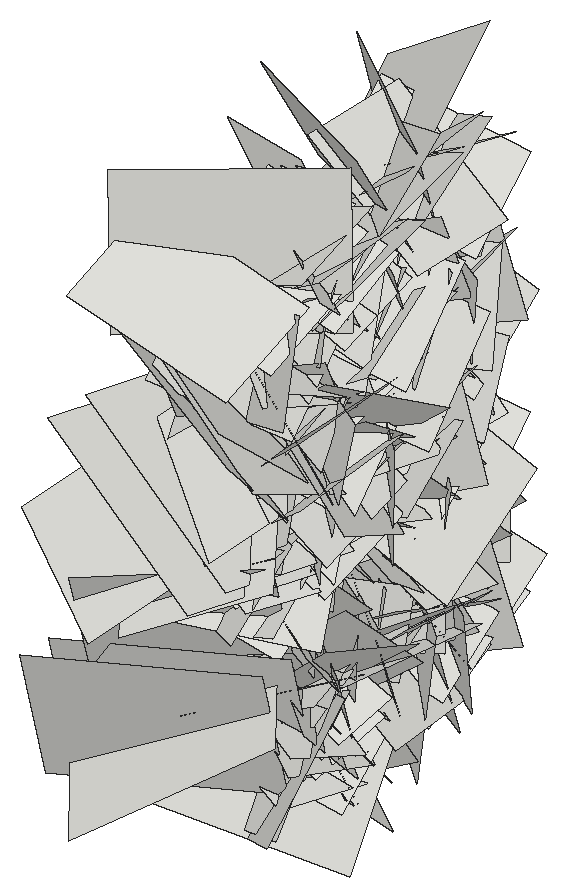
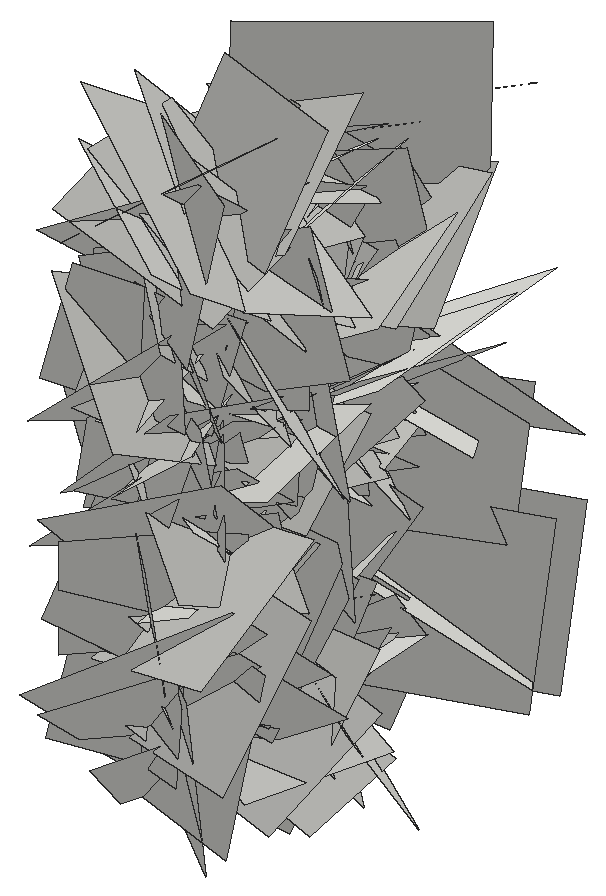
# SketchUp Ruby script. Lengths in inches.
U = 1.inch
M = Sketchup.active_model
def pt(a) = Geom::Point3d.new(a.map { |v| v * U })
def face(e, loops, mat)
  f = e.add_face(loops[0].map { |a| pt(a) })
  loops[1..].each { |l| e.add_face(l.map { |a| pt(a) }).erase! }
  f.material = f.back_material = mat if mat
  f
end
# faces: each face lists its corners as indices into pts; further lists are holes
def faces(e, pts, list, mat = nil) = list.each { |f| face(e, (f[0].is_a?(Array) ? f : [f]).map { |l| l.map { |i| pts[i] } }, mat) }
# xy, xz, yz: faces in a plane at the given z, y or x. An outline is a flat list of corners, or four numbers for a rectangle; further outlines are holes
def ring(l) = l.size == 4 ? [[l[0], l[1]], [l[2], l[1]], [l[2], l[3]], [l[0], l[3]]] : l.each_slice(2).to_a
def flat(e, list, mat, &to3) = list.each { |f| face(e, (f[0].is_a?(Array) ? f : [f]).map { |l| ring(l).map { |u, v| to3.(u, v) } }, mat) }
def xy(e, z, list, mat = nil) = flat(e, list, mat) { |x, y| [x, y, z] }
def xz(e, y, list, mat = nil) = flat(e, list, mat) { |x, z| [x, y, z] }
def yz(e, x, list, mat = nil) = flat(e, list, mat) { |y, z| [x, y, z] }
def lines(e, pts, list) = list.each { |a, b| e.add_line(pt(pts[a]), pt(pts[b])) }
# prism: a flat outline (further loops are holes) pulled along v
def prism(e, loops, v, mat = nil)
  f = face(e, loops, mat); d = Geom::Vector3d.new(v.map { |x| x * U })
  f.pushpull(f.normal.samedirection?(d) ? d.length : -d.length)
end
def box(e, o, s, mat = nil) = prism(e, [[o, [o[0] + s[0], o[1], o[2]], [o[0] + s[0], o[1] + s[1], o[2]], [o[0], o[1] + s[1], o[2]]]], [0, 0, s[2]], mat)
def at(x, y, z, deg = 0) = Geom::Transformation.translation(pt([x, y, z])) * Geom::Transformation.rotation(ORIGIN, Z_AXIS, deg.degrees)
def axes(o, x, y, z) = Geom::Transformation.new([*x, 0, *y, 0, *z, 0, *pt(o).to_a, 1])
def part(name) = M.definitions.add(name)
# library, detail: a bought-in or finely detailed component or shape, given as its bounding box
def library(name, o, s) = part(name).tap { |d| box(d.entities, o, s) }
def detail(e, o, s) = box(e.add_group.entities, o, s)
def put(e, d, t, mat = nil) = e.add_instance(d, t).tap { |i| i.material = mat if mat }
def group(e, t, mat = nil) = e.add_group.tap { |g| g.transformation = t; g.material = mat if mat }.entities
root = M.entities
c1 = part("Component\#6")
p = [[0.01,0,0],[0,3.24,4.54],[4.32,3.24,4.54],[4.33,0,0]]
faces(c1.entities,p,[[0,1,2,3]])
put(root,c1,axes([404.99,125.5,13.2],[-1.07209,0.56535,0.5401],[-0.40295,0.41611,-1.14744],[-0.72423,-1.06841,-0.1611]))
put(root,c1,axes([404.88,125.3125,7.6875],[-0.15543,0.49215,-1.26812],[-0.29157,-1.25984,-0.45713],[-1.41209,0.20597,0.23397]))
put(root,c1,axes([404.88,126.76,7.6875],[-0.15543,0.49215,-1.26812],[-0.29157,-1.25984,-0.45713],[-1.41209,0.20597,0.23397]))
put(root,c1,axes([404.88,135.96,3.29],[-0.1622,-0.76384,1.11136],[-0.23079,1.11781,0.7383],[-1.4107,-0.09505,-0.24857]))
put(root,c1,axes([404.88,130.15,15.41],[-0.24379,0.89731,1.03665],[-0.02149,1.04879,-0.91232],[-1.45316,-0.16605,-0.16042]))
put(root,c1,axes([404.88,136.82,5.83],[-0.1656,-1.02965,0.80161],[-0.14776,0.81588,1.02082],[-1.37528,0.03632,-0.2062]))
put(root,c1,axes([404.88,130.78,10.54],[-0.24762,-1.26357,-0.1726],[0.00687,-0.17664,1.28442],[-1.3518,0.23056,0.03815]))
put(root,c1,axes([406.05,124.5,5.79],[-0.83668,1.07369,0.2523],[-0.21003,0.16716,-1.33127],[-1.15009,-0.81162,0.05958]))
put(root,c1,axes([404.88,138.98,4.78],[-0.22268,-0.9196,-0.8307],[-0.07298,-0.83259,0.9391],[-1.31157,0.20246,0.08879]))
put(root,c1,axes([404.88,128.0625,10.23],[-0.10909,-1.3698,0.20566],[0.00727,0.20572,1.37363],[-1.46824,0.1028,-0.00848]))
put(root,c1,axes([404.88,129.98,10.23],[-0.10909,-1.3698,0.20566],[0.00727,0.20572,1.37363],[-1.46824,0.1028,-0.00848]))
put(root,c1,axes([404.88,135.39,1.18],[-0.01455,-0.40823,1.27358],[-0.1801,1.26386,0.40328],[-1.40617,-0.15765,-0.06483]))
put(root,c1,axes([404.88,137,19.49],[-0.23927,-0.1296,-1.18474],[-0.04055,-1.20439,0.13904],[-1.26266,0.06324,0.22004]))
put(root,c1,axes([404.88,127.67,13.74],[-0.06329,-0.97705,0.81505],[-0.12838,0.8166,0.97005],[-1.34259,-0.03203,-0.13118]))
put(root,c1,axes([404.88,125.99,1.35],[-0.00241,0.79041,1.08039],[-0.06651,1.07914,-0.78963],[-1.41741,-0.05198,0.03522]))
put(root,c1,axes([404.88,132.12,7.08],[0.00585,1.22451,-0.43101],[-0.11167,-0.42917,-1.22063],[-1.3715,0.04016,0.09755]))
put(root,c1,axes([404.88,133.15,22.79],[-0.15509,1.06813,0.73269],[0.10614,0.74447,-1.06531],[-1.36888,-0.06329,-0.16562]))
put(root,c1,axes([404.88,128.24,17.68],[-0.22785,0.52614,1.07761],[0.06777,1.09826,-0.52347],[-1.26934,-0.03581,-0.22138]))
put(root,c1,axes([404.88,133.04,19.75],[-0.14526,-0.49923,0.95494],[-0.24012,0.95446,0.46647],[-1.11669,-0.1403,-0.22453]))
put(root,c1,axes([404.88,139.8125,5.82],[-0.12038,-0.94885,-0.86303],[0.08352,-0.86993,0.94607],[-1.35702,0.03063,0.13479]))
put(root,c1,axes([404.88,131.95,0.87],[-0.07095,-0.70744,0.83659],[-0.30432,0.82019,0.6706],[-1.12076,-0.17792,-0.23504]))
put(root,c1,axes([404.88,125.82,11.42],[-0.20547,0.4933,-0.99975],[-0.03886,-1.01702,-0.49472],[-1.18108,-0.05236,0.1902]))
put(root,c1,axes([404.88,129.66,12.47],[0.1081,-1.2535,0.58167],[0.00417,0.58351,1.25678],[-1.46479,-0.09085,0.0465]))
put(root,c1,axes([404.88,129.48,20.64],[0.14207,1.22324,0.51937],[-0.11373,0.53026,-1.2212],[-1.40407,0.08082,0.15147]))
put(root,c1,axes([404.88,134.94,17.85],[-0.08672,-0.29938,1.1859],[0.04442,1.18717,0.30259],[-1.29573,0.06074,-0.069]))
put(root,c1,axes([404.88,133.96,9.66],[-0.06967,-1.04066,0.34132],[-0.1454,0.34706,1.03175],[-1.15177,0.01914,-0.15089]))
put(root,c1,axes([404.88,126.61,12.8],[0.1414,-0.87971,0.87765],[-0.19082,0.8597,0.88908],[-1.30331,-0.22132,-0.03495]))
put(root,c1,axes([404.88,129.42,5.47],[0.26825,1.30607,0.06413],[-0.25565,0.11082,-1.30519],[-1.36232,0.23638,0.25756]))
put(root,c1,axes([404.88,136.29,19.65],[-0.239,0.33681,-1.04778],[0.13934,-1.05364,-0.36698],[-1.15826,-0.19625,0.17205]))
put(root,c1,axes([404.88,131.16,1.32],[-0.11103,-1.00768,0.14491],[-0.13016,0.15712,1.00381],[-1.07125,0.08535,-0.13699]))
put(root,c1,axes([404.88,129.81,24.32],[0.08615,-0.07511,-1.33483],[0.12267,-1.33188,0.08199],[-1.41184,-0.12031,-0.07433]))
put(root,c1,axes([400.91,129.35,18.22],[-0.07955,-0.40219,0.442],[-0.06566,0.44831,0.39741],[0.63004,-0.00406,0.09723]))
put(root,c1,axes([404.88,127.69,20.12],[0.02742,-1.01137,-0.35231],[-0.21232,-0.35076,0.99222],[-1.1152,0.04191,-0.19757]))
put(root,c1,axes([404.88,130,20.12],[0.02742,-1.01137,-0.35231],[-0.21232,-0.35076,0.99222],[-1.1152,0.04191,-0.19757]))
put(root,c1,axes([400.91,138.1,17.99],[-0.00934,-0.49027,-0.41508],[-0.1892,-0.3969,0.47259],[0.65411,-0.1218,0.13076]))
put(root,c1,axes([404.88,127.92,6.47],[0.03611,0.05394,1.13531],[-0.09971,1.13206,-0.05096],[-1.20066,-0.09239,0.03838]))
put(root,c1,axes([405.6,124.93,11.12],[-0.54058,0.75668,0.32998],[-0.30141,0.20311,-0.90522],[-0.82148,-0.57246,0.11499]))
put(root,c1,axes([404.88,134.14,22.88],[-0.03825,0.99518,-0.25742],[-0.13842,-0.25993,-0.98657],[-1.08078,-0.00193,0.13547]))
put(root,c1,axes([400.91,134.77,2.57],[-0.05447,0.40704,0.46107],[-0.08155,0.45478,-0.41007],[0.64681,0.09162,-0.01288]))
put(root,c1,axes([404.88,131.18,15.16],[-0.15294,-1.16278,0.39158],[0.28955,0.35393,1.15166],[-1.26792,0.22109,0.21577]))
put(root,c1,axes([404.88,131.94,16.85],[0.08825,-0.96476,0.81898],[0.08011,0.82307,0.9619],[-1.33903,-0.01434,0.11152]))
put(root,c1,axes([404.88,128.56,10.3125],[0.23413,0.04823,1.24691],[-0.1221,1.26168,-0.02839],[-1.31707,-0.10839,0.22429]))
put(root,c1,axes([404.88,133.91,11.1875],[0.02059,0.92356,-0.8814],[0.20413,-0.87353,-0.91107],[-1.33776,-0.11908,-0.15259]))
put(root,c1,axes([404.88,130.99,8.6],[-0.04494,-0.64922,0.68663],[-0.20873,0.6783,0.62918],[-0.97967,-0.11474,-0.16555]))
put(root,c1,axes([404.88,129.625,19.87],[0.14331,0.9196,0.97349],[0.15794,0.96203,-0.92947],[-1.41069,0.20113,-0.00516]))
put(root,c1,axes([404.88,137.87,11.82],[-0.23548,-0.98581,-0.19043],[0.17104,-0.22756,0.98976],[-1.05044,0.18394,0.20385]))
put(root,c1,axes([400.91,131.8,8.64],[-0.08497,0.05507,0.67491],[-0.04101,0.67814,-0.05993],[0.71661,0.04534,0.0766]))
put(root,c1,axes([404.88,134.95,12.42],[-0.03363,0.92541,-1.00089],[0.39451,-0.95725,-0.89685],[-1.39004,-0.29406,-0.23032]))
put(root,c1,axes([400.91,131.9,7.66],[-0.03371,0.19161,0.61883],[-0.06203,0.6162,-0.1938],[0.68388,0.06533,0.01292]))
put(root,c1,axes([404.88,131.74,20.5625],[0.11289,-0.41624,-1.03402],[-0.06809,-1.03929,0.41174],[-1.17957,0.02016,-0.12272]))
put(root,c1,axes([404.88,138.97,11.375],[0.02639,-0.72989,-0.72722],[-0.07911,-0.7268,0.72691],[-1.08928,0.0351,-0.07041]))
put(root,c1,axes([404.88,128.87,2.92],[-0.01411,0.95221,-0.19006],[-0.11482,-0.19035,-0.94606],[-1.02282,0.00823,0.10882]))
put(root,c1,axes([400.91,134.26,15.51],[-0.13639,0.72841,-0.25059],[-0.07067,-0.26364,-0.7321],[0.81346,0.09922,-0.10562]))
put(root,c1,axes([404.88,129.68,16.21],[-0.16446,-0.17941,-0.82447],[-0.07006,-0.83314,0.19373],[-0.89165,0.09856,0.13685]))
put(root,c1,axes([400.91,127.28,0.51],[-0.04452,-0.40985,0.5808],[-0.07759,0.58122,0.40485],[0.7495,0.03582,0.07641]))
put(root,c1,axes([404.88,133.2,0.29],[0.16868,0.00753,1.30134],[0.16064,1.302,-0.02607],[-1.37005,0.15359,0.15716]))
put(root,c1,axes([400.91,134.57,7.51],[-0.06425,-0.0713,-0.65597],[0.02618,-0.65852,0.06929],[0.69893,0.01811,-0.0629]))
put(root,c1,axes([404.88,128.52,17.74],[-0.08604,0.43028,-0.81229],[-0.04293,-0.81633,-0.42838],[-0.97342,-0.00203,0.0907]))
put(root,c1,axes([400.91,132.11,13.83],[-0.12823,-0.67114,-0.46171],[-0.10246,-0.45164,0.68184],[0.85739,-0.15435,0.01243]))
put(root,c1,axes([404.88,133.79,15.82],[-0.11741,-0.82822,-0.37202],[-0.00882,-0.37384,0.83474],[-0.96237,0.10447,0.03774]))
put(root,c1,axes([400.91,131.53,3.64],[-0.03356,0.34972,-0.55611],[0.01458,-0.55628,-0.35061],[0.69619,0.02851,-0.01946]))
put(root,c1,axes([400.91,130.57,14.69],[-0.08088,0.56373,-0.36339],[0.06437,-0.35843,-0.56878],[0.70803,0.09698,0.0102]))
put(root,c1,axes([404.88,130.125,12.36],[0.14413,1.23778,0.56401],[0.30073,0.52855,-1.22835],[-1.41013,0.23923,-0.20431]))
put(root,c1,axes([404.88,129.28,18.375],[-0.15104,-0.37703,-0.77667],[0.00911,-0.78776,0.38083],[-0.9151,0.05438,0.13199]))
put(root,c1,axes([404.88,132.6,22.9],[-0.05818,0.99288,0.05669],[0.07779,0.06066,-0.99145],[-1.05129,-0.05046,-0.07649]))
put(root,c1,axes([400.91,133.3125,17.59],[0.01529,0.27468,0.5349],[0.08187,0.52978,-0.27413],[0.6321,-0.07526,0.02257]))
put(root,c1,axes([400.91,129.84,16.13],[0.05288,0.68465,0.04631],[-0.09068,0.05228,-0.68068],[0.72171,-0.04359,-0.08892]))
put(root,c1,axes([404.88,129.45,15.69],[0.00555,0.72683,0.86308],[0.19522,0.85097,-0.71774],[-1.18002,0.1442,-0.11468]))
put(root,c1,axes([400.91,129.41,10.95],[-0.18775,-0.48629,-0.69123],[0.00245,-0.70652,0.49646],[0.89586,-0.09998,-0.14623]))
put(root,c1,axes([400.91,132.63,6.14],[-0.10731,0.87556,-0.00554],[-0.12201,-0.01884,-0.87366],[0.92006,0.09962,-0.1165]))
put(root,c1,axes([404.88,133.96,12.5],[-0.03937,0.24323,0.81298],[-0.12274,0.80469,-0.24604],[-0.89109,-0.12158,-0.00203]))
put(root,c1,axes([404.88,127.6,6.32],[-0.09105,0.77875,-0.27248],[-0.08108,-0.28029,-0.77696],[-0.87078,-0.05533,0.10084]))
put(root,c1,axes([404.88,133.1,9.3125],[0.02086,0.87239,-0.16813],[-0.14049,-0.16341,-0.8634],[-0.93122,0.04419,0.12649]))
put(root,c1,axes([404.88,131.05,1.96],[0.03915,-1.05631,0.36623],[0.17317,0.36759,1.04378],[-1.17236,0.01903,0.16641]))
put(root,c1,axes([400.91,133.88,6.93],[-0.12434,-0.60409,0.41763],[0.12699,0.40152,0.61444],[0.76804,-0.16419,-0.03398]))
put(root,c1,axes([404.88,136.93,7.59],[0.11136,0.24127,-0.97313],[-0.07388,-0.97433,-0.24909],[-1.06018,0.09324,-0.08486]))
put(root,c1,axes([400.91,130.03,2.94],[-0.11679,-0.3481,0.76621],[-0.04914,0.77408,0.34502],[0.89071,-0.00294,0.1195]))
put(root,c1,axes([400.91,129.23,5.41],[-0.17398,-0.60139,0.60701],[0.02487,0.6147,0.61536],[0.9054,-0.13245,0.09973]))
put(root,c1,axes([404.88,132.5,3.06],[0.12033,-0.77552,-0.96336],[0.26418,-0.93322,0.78062],[-1.28404,-0.26468,0.07033]))
put(root,c1,axes([400.91,129.18,10.77],[0.08644,0.04023,-0.60323],[0.06997,-0.60565,-0.03147],[0.63702,0.06107,0.08531]))
put(root,c1,axes([404.88,132.55,10.48],[0.11298,-1.07137,-0.22101],[0.09706,-0.21254,1.07447],[-1.1555,-0.12261,0.06864]))
put(root,c1,axes([400.91,128.34,18.92],[0.04874,0.38349,0.62334],[-0.06251,0.62448,-0.37984],[0.77325,0.02631,-0.07]))
put(root,c1,axes([400.91,129.8,15.91],[0.05085,-0.71724,0.33006],[-0.13843,0.31891,0.71198],[0.82538,0.09767,0.09907]))
put(root,c1,axes([404.88,127.86,19.19],[0.25173,1.01088,0.57921],[0.04385,0.58343,-1.03521],[-1.23418,0.22691,0.08136]))
put(root,c1,axes([404.88,127.34,21.1],[0.03089,0.79811,0.32897],[-0.11706,0.3299,-0.79059],[-0.90753,-0.01539,0.11317]))
put(root,c1,axes([400.91,133.42,16.97],[-0.14677,0.94615,0.46149],[-0.22557,0.4307,-0.94687],[1.09283,0.21597,-0.13346]))
put(root,c1,axes([400.91,133.96,6.46],[-0.0893,0.11056,0.97068],[-0.19494,0.95507,-0.12474],[1.01706,0.19277,0.06132]))
put(root,c1,axes([404.88,136.53,11.26],[0.01536,-0.64622,-0.54667],[-0.11065,-0.54394,0.64022],[-0.89037,0.05645,-0.089]))
put(root,c1,axes([400.91,131.99,-0.9375],[0.0225,-0.54484,0.50649],[-0.02225,0.50605,0.54525],[0.78821,0.02984,0.00093]))
put(root,c1,axes([404.88,127.95,5.4],[-0.05879,0.74539,0.22064],[-0.10629,0.21249,-0.74307],[-0.81711,-0.08127,0.08079]))
put(root,c1,axes([400.91,125.86,8.82],[0.02658,0.53015,0.39509],[0.11889,0.38623,-0.52538],[0.69069,-0.08688,0.07523]))
put(root,c1,axes([400.91,131.86,3.01],[0.01467,-0.55248,-0.51034],[-0.00827,-0.51051,0.55244],[0.7972,0.00487,0.01512]))
put(root,c1,axes([400.91,136.82,15.87],[-0.16772,-0.74319,-0.48228],[0.03783,-0.49486,0.75087],[0.93836,-0.11289,-0.11647]))
put(root,c1,axes([404.88,125.93,11.7],[-0.16945,0.67455,-0.05214],[-0.09647,-0.07453,-0.68517],[-0.71064,-0.15073,0.10544]))
put(root,c1,axes([404.88,127.92,4.7],[-0.092,0.70183,0.2556],[-0.07294,0.24871,-0.70628],[-0.78837,-0.10491,0.03552]))
put(root,c1,axes([404.88,128.53,16.93],[0.30517,1.08519,-0.55956],[0.1011,-0.59314,-1.10124],[-1.29027,0.21019,-0.21864]))
put(root,c1,axes([400.91,137.37,4.77],[-0.01509,-0.67708,-0.46908],[-0.05072,-0.46768,0.67651],[0.87164,-0.03894,0.03124]))
put(root,c1,axes([404.88,133.14,16.06],[0.03738,-0.31853,0.81486],[-0.04959,0.81367,0.32009],[-0.92608,-0.05642,0.01575]))
put(root,c1,axes([404.88,133.58,20.74],[0.06025,0.71815,0.57437],[0.00066,0.57544,-0.71955],[-0.97476,0.04478,0.03501]))
put(root,c1,axes([404.88,131.35,15.19],[-0.02447,0.82058,-0.14823],[-0.01236,-0.14859,-0.82075],[-0.8838,-0.02064,0.01558]))
put(root,c1,axes([400.91,130.01,4.69],[0.05447,0.12092,0.77662],[-0.06993,0.77619,-0.11649],[0.83019,0.05744,-0.06077]))
put(root,c1,axes([404.88,135.14,15.06],[0.15738,0.18416,-1.10832],[0.16264,-1.1108,-0.16402],[-1.17977,-0.12857,-0.17046]))
put(root,c1,axes([404.88,133.07,14.74],[0.12706,0.28525,0.91315],[-0.02767,0.92092,-0.28425],[-1.01369,0.01061,0.12222]))
put(root,c1,axes([404.88,132.96,18.89],[0.10145,-0.91774,-0.17179],[-0.02227,-0.17476,0.92192],[-0.98945,-0.09016,-0.03837]))
put(root,c1,axes([400.91,135.65,2.32],[-0.1935,-1.06071,0.09437],[-0.13048,0.11613,1.0671],[1.12123,-0.16954,0.14047]))
put(root,c1,axes([400.91,136.42,13.64],[0.14309,-0.55174,0.41683],[-0.03038,0.41987,0.56505],[0.73236,0.12522,-0.058]))
put(root,c1,axes([404.88,137.27,19.36],[0.1763,0.15017,-0.9005],[-0.15684,-0.89878,-0.17721],[-0.95491,0.17535,-0.13715]))
put(root,c1,axes([404.88,130.2,1.79],[0.1042,-0.77086,0.73803],[0.17604,0.74317,0.75412],[-1.11745,0.04519,0.18762]))
put(root,c1,axes([404.88,136.01,11.51],[-0.06598,-0.27091,0.62957],[-0.16839,0.62065,0.25136],[-0.70672,-0.12259,-0.11867]))
put(root,c1,axes([400.91,133.51,8.98],[-0.15319,0.47062,-0.90401],[-0.09722,-0.91536,-0.46187],[1.07594,-0.0157,-0.17044]))
put(root,c1,axes([404.88,126.24,11.02],[-0.17433,0.41563,0.4957],[-0.04437,0.50356,-0.43611],[-0.68427,-0.13854,-0.09801]))
put(root,c1,axes([400.91,132.67,11.61],[-0.16439,-1.14375,-0.17253],[-0.24163,-0.14044,1.13591],[1.20204,-0.18465,0.20475]))
put(root,c1,axes([404.88,132.67,11.61],[0.16439,-1.14375,-0.17253],[0.24163,-0.14044,1.13591],[-1.20204,-0.18465,0.20475]))
put(root,c1,axes([400.91,126.24,11.02],[0.17433,0.41563,0.4957],[0.04437,0.50356,-0.43611],[0.68427,-0.13854,-0.09801]))
put(root,c1,axes([404.88,133.51,8.98],[0.15319,0.47062,-0.90401],[0.09722,-0.91536,-0.46187],[-1.07594,-0.0157,-0.17044]))
put(root,c1,axes([400.91,136.01,11.51],[0.06598,-0.27091,0.62957],[0.16839,0.62065,0.25136],[0.70672,-0.12259,-0.11867]))
put(root,c1,axes([400.91,130.2,1.79],[-0.1042,-0.77086,0.73803],[-0.17604,0.74317,0.75412],[1.11745,0.04519,0.18762]))
put(root,c1,axes([400.91,137.27,19.36],[-0.1763,0.15017,-0.9005],[0.15684,-0.89878,-0.17721],[0.95491,0.17535,-0.13715]))
put(root,c1,axes([404.88,136.42,13.64],[-0.14309,-0.55174,0.41683],[0.03038,0.41987,0.56505],[-0.73236,0.12522,-0.058]))
put(root,c1,axes([404.88,135.65,2.32],[0.1935,-1.06071,0.09437],[0.13048,0.11613,1.0671],[-1.12123,-0.16954,0.14047]))
put(root,c1,axes([400.91,132.96,18.89],[-0.10145,-0.91774,-0.17179],[0.02227,-0.17476,0.92192],[0.98945,-0.09016,-0.03837]))
put(root,c1,axes([400.91,133.07,14.74],[-0.12706,0.28525,0.91315],[0.02767,0.92092,-0.28425],[1.01369,0.01061,0.12222]))
put(root,c1,axes([400.91,135.14,15.06],[-0.15738,0.18416,-1.10832],[-0.16264,-1.1108,-0.16402],[1.17977,-0.12857,-0.17046]))
put(root,c1,axes([404.88,130.01,4.69],[-0.05447,0.12092,0.77662],[0.06993,0.77619,-0.11649],[-0.83019,0.05744,-0.06077]))
put(root,c1,axes([400.91,131.35,15.19],[0.02447,0.82058,-0.14823],[0.01236,-0.14859,-0.82075],[0.8838,-0.02064,0.01558]))
put(root,c1,axes([400.91,133.58,20.74],[-0.06025,0.71815,0.57437],[-0.00066,0.57544,-0.71955],[0.97476,0.04478,0.03501]))
put(root,c1,axes([400.91,133.14,16.06],[-0.03738,-0.31853,0.81486],[0.04959,0.81367,0.32009],[0.92608,-0.05642,0.01575]))
put(root,c1,axes([404.88,137.37,4.77],[0.01509,-0.67708,-0.46908],[0.05072,-0.46768,0.67651],[-0.87164,-0.03894,0.03124]))
put(root,c1,axes([400.91,128.53,16.93],[-0.30517,1.08519,-0.55956],[-0.1011,-0.59314,-1.10124],[1.29027,0.21019,-0.21864]))
put(root,c1,axes([400.91,127.92,4.7],[0.092,0.70183,0.2556],[0.07294,0.24871,-0.70628],[0.78837,-0.10491,0.03552]))
put(root,c1,axes([400.91,125.93,11.7],[0.16945,0.67455,-0.05214],[0.09647,-0.07453,-0.68517],[0.71064,-0.15073,0.10544]))
put(root,c1,axes([404.88,136.82,15.87],[0.16772,-0.74319,-0.48228],[-0.03783,-0.49486,0.75087],[-0.93836,-0.11289,-0.11647]))
put(root,c1,axes([404.88,131.86,3.01],[-0.01467,-0.55248,-0.51034],[0.00827,-0.51051,0.55244],[-0.7972,0.00487,0.01512]))
put(root,c1,axes([404.88,125.86,8.82],[-0.02658,0.53015,0.39509],[-0.11889,0.38623,-0.52538],[-0.69069,-0.08688,0.07523]))
put(root,c1,axes([400.91,127.95,5.4],[0.05879,0.74539,0.22064],[0.10629,0.21249,-0.74307],[0.81711,-0.08127,0.08079]))
put(root,c1,axes([404.88,131.99,-0.9375],[-0.0225,-0.54484,0.50649],[0.02225,0.50605,0.54525],[-0.78821,0.02984,0.00093]))
put(root,c1,axes([400.91,136.53,11.26],[-0.01536,-0.64622,-0.54667],[0.11065,-0.54394,0.64022],[0.89037,0.05645,-0.089]))
put(root,c1,axes([404.88,133.96,6.46],[0.0893,0.11056,0.97068],[0.19494,0.95507,-0.12474],[-1.01706,0.19277,0.06132]))
put(root,c1,axes([404.88,133.42,16.97],[0.14677,0.94615,0.46149],[0.22557,0.4307,-0.94687],[-1.09283,0.21597,-0.13346]))
put(root,c1,axes([400.91,127.34,21.1],[-0.03089,0.79811,0.32897],[0.11706,0.3299,-0.79059],[0.90753,-0.01539,0.11317]))
put(root,c1,axes([400.91,127.86,19.19],[-0.25173,1.01088,0.57921],[-0.04385,0.58343,-1.03521],[1.23418,0.22691,0.08136]))
put(root,c1,axes([404.88,129.8,15.91],[-0.05085,-0.71724,0.33006],[0.13843,0.31891,0.71198],[-0.82538,0.09767,0.09907]))
put(root,c1,axes([404.88,128.34,18.92],[-0.04874,0.38349,0.62334],[0.06251,0.62448,-0.37984],[-0.77325,0.02631,-0.07]))
put(root,c1,axes([400.91,132.55,10.48],[-0.11298,-1.07137,-0.22101],[-0.09706,-0.21254,1.07447],[1.1555,-0.12261,0.06864]))
put(root,c1,axes([404.88,129.18,10.77],[-0.08644,0.04023,-0.60323],[-0.06997,-0.60565,-0.03147],[-0.63702,0.06107,0.08531]))
put(root,c1,axes([400.91,132.5,3.06],[-0.12033,-0.77552,-0.96336],[-0.26418,-0.93322,0.78062],[1.28404,-0.26468,0.07033]))
put(root,c1,axes([404.88,129.23,5.41],[0.17398,-0.60139,0.60701],[-0.02487,0.6147,0.61536],[-0.9054,-0.13245,0.09973]))
put(root,c1,axes([404.88,130.03,2.94],[0.11679,-0.3481,0.76621],[0.04914,0.77408,0.34502],[-0.89071,-0.00294,0.1195]))
put(root,c1,axes([400.91,136.93,7.59],[-0.11136,0.24127,-0.97313],[0.07388,-0.97433,-0.24909],[1.06018,0.09324,-0.08486]))
put(root,c1,axes([404.88,133.88,6.93],[0.12434,-0.60409,0.41763],[-0.12699,0.40152,0.61444],[-0.76804,-0.16419,-0.03398]))
put(root,c1,axes([400.91,131.05,1.96],[-0.03915,-1.05631,0.36623],[-0.17317,0.36759,1.04378],[1.17236,0.01903,0.16641]))
put(root,c1,axes([400.91,133.1,9.3125],[-0.02086,0.87239,-0.16813],[0.14049,-0.16341,-0.8634],[0.93122,0.04419,0.12649]))
put(root,c1,axes([400.91,127.6,6.32],[0.09105,0.77875,-0.27248],[0.08108,-0.28029,-0.77696],[0.87078,-0.05533,0.10084]))
put(root,c1,axes([400.91,133.96,12.5],[0.03937,0.24323,0.81298],[0.12274,0.80469,-0.24604],[0.89109,-0.12158,-0.00203]))
put(root,c1,axes([404.88,132.63,6.14],[0.10731,0.87556,-0.00554],[0.12201,-0.01884,-0.87366],[-0.92006,0.09962,-0.1165]))
put(root,c1,axes([404.88,129.41,10.95],[0.18775,-0.48629,-0.69123],[-0.00245,-0.70652,0.49646],[-0.89586,-0.09998,-0.14623]))
put(root,c1,axes([400.91,129.45,15.69],[-0.00555,0.72683,0.86308],[-0.19522,0.85097,-0.71774],[1.18002,0.1442,-0.11468]))
put(root,c1,axes([404.88,129.84,16.13],[-0.05288,0.68465,0.04631],[0.09068,0.05228,-0.68068],[-0.72171,-0.04359,-0.08892]))
put(root,c1,axes([404.88,133.3125,17.59],[-0.01529,0.27468,0.5349],[-0.08187,0.52978,-0.27413],[-0.6321,-0.07526,0.02257]))
put(root,c1,axes([400.91,132.6,22.9],[0.05818,0.99288,0.05669],[-0.07779,0.06066,-0.99145],[1.05129,-0.05046,-0.07649]))
put(root,c1,axes([400.91,129.28,18.375],[0.15104,-0.37703,-0.77667],[-0.00911,-0.78776,0.38083],[0.9151,0.05438,0.13199]))
put(root,c1,axes([400.91,130.125,12.36],[-0.14413,1.23778,0.56401],[-0.30073,0.52855,-1.22835],[1.41013,0.23923,-0.20431]))
put(root,c1,axes([404.88,130.57,14.69],[0.08088,0.56373,-0.36339],[-0.06437,-0.35843,-0.56878],[-0.70803,0.09698,0.0102]))
put(root,c1,axes([404.88,131.53,3.64],[0.03356,0.34972,-0.55611],[-0.01458,-0.55628,-0.35061],[-0.69619,0.02851,-0.01946]))
put(root,c1,axes([400.91,133.79,15.82],[0.11741,-0.82822,-0.37202],[0.00882,-0.37384,0.83474],[0.96237,0.10447,0.03774]))
put(root,c1,axes([404.88,132.11,13.83],[0.12823,-0.67114,-0.46171],[0.10246,-0.45164,0.68184],[-0.85739,-0.15435,0.01243]))
put(root,c1,axes([400.91,128.52,17.74],[0.08604,0.43028,-0.81229],[0.04293,-0.81633,-0.42838],[0.97342,-0.00203,0.0907]))
put(root,c1,axes([404.88,134.57,7.51],[0.06425,-0.0713,-0.65597],[-0.02618,-0.65852,0.06929],[-0.69893,0.01811,-0.0629]))
